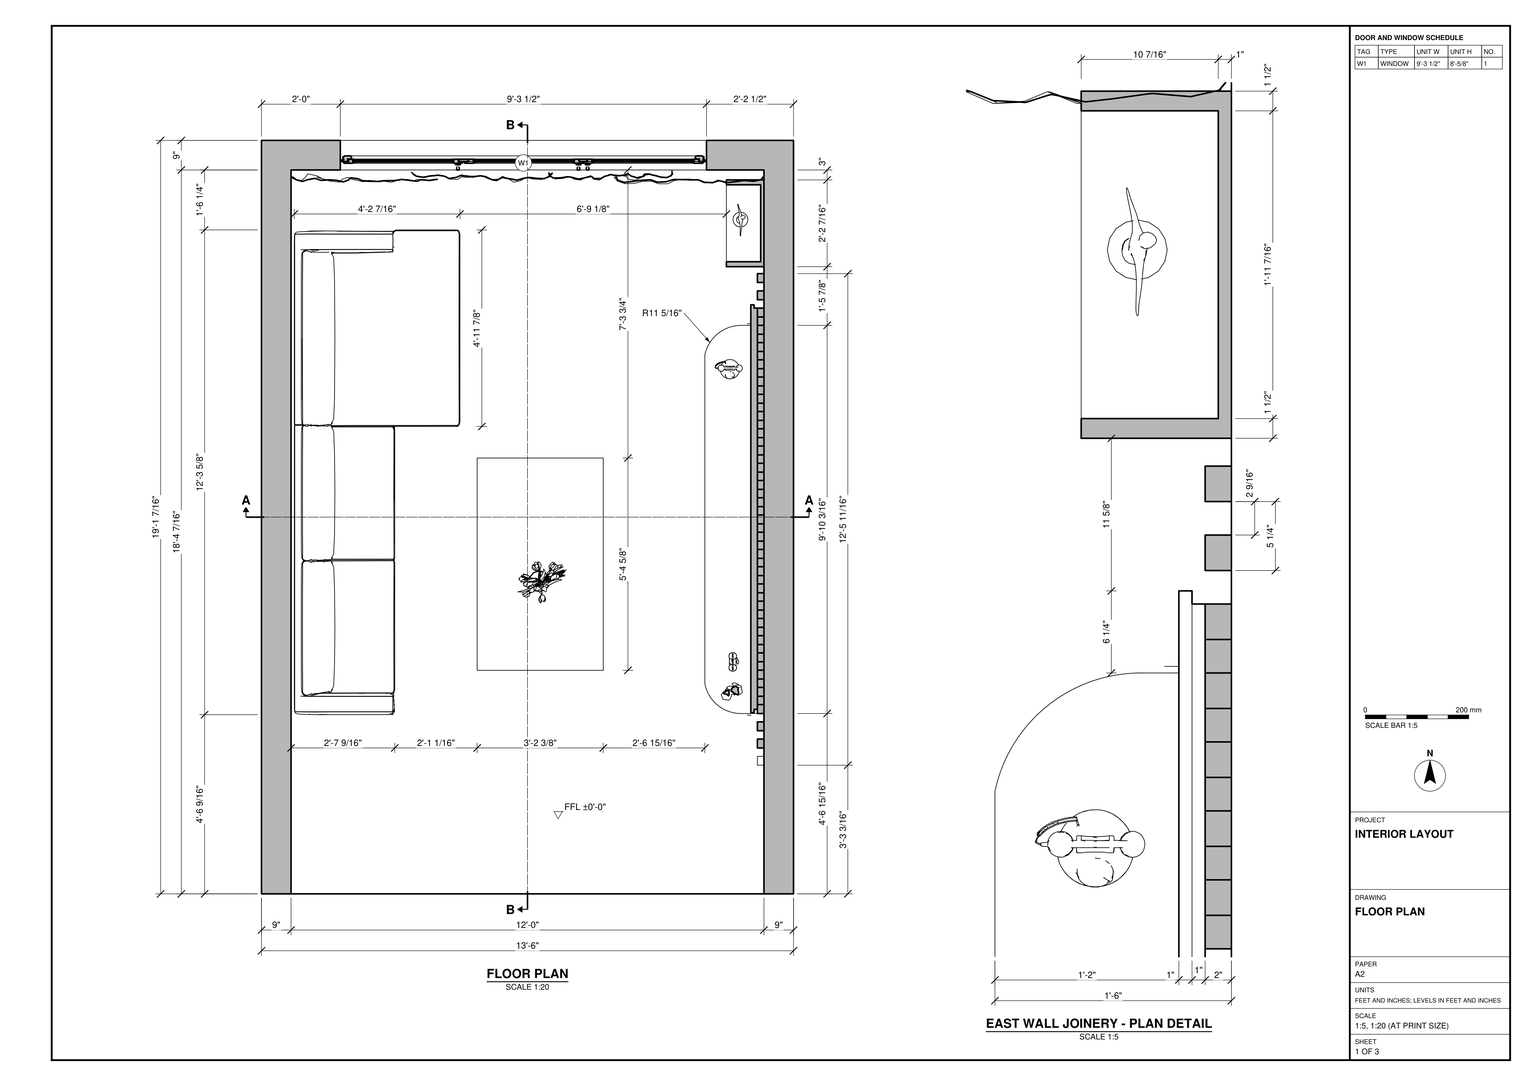
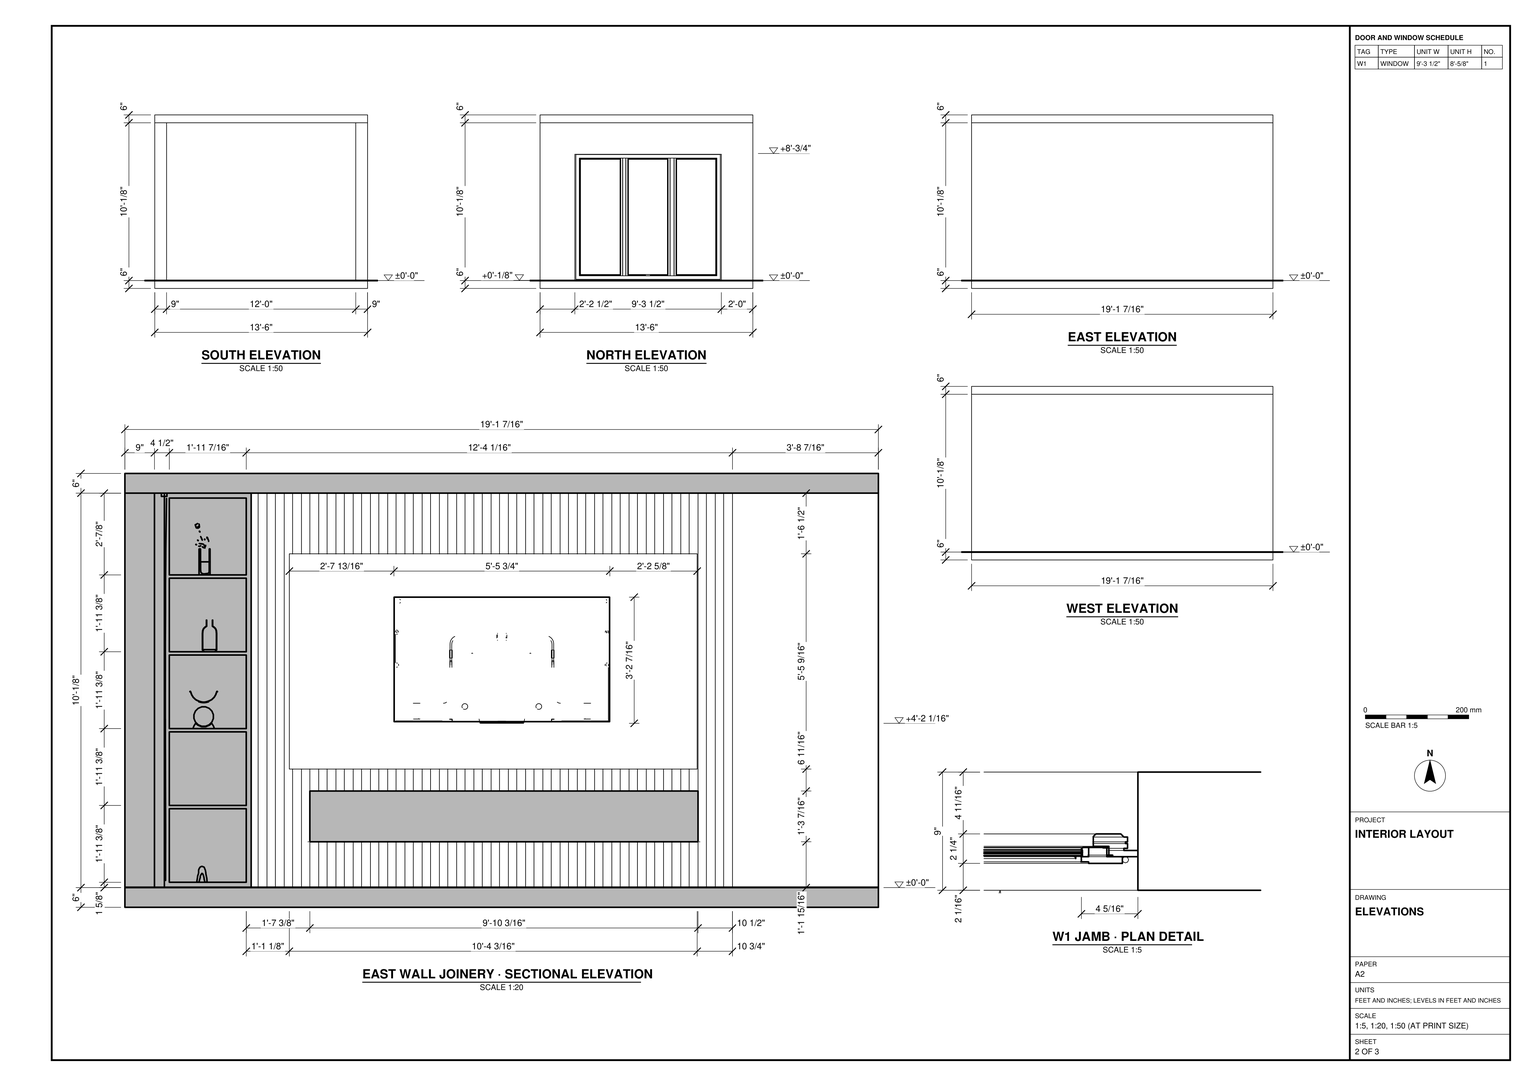
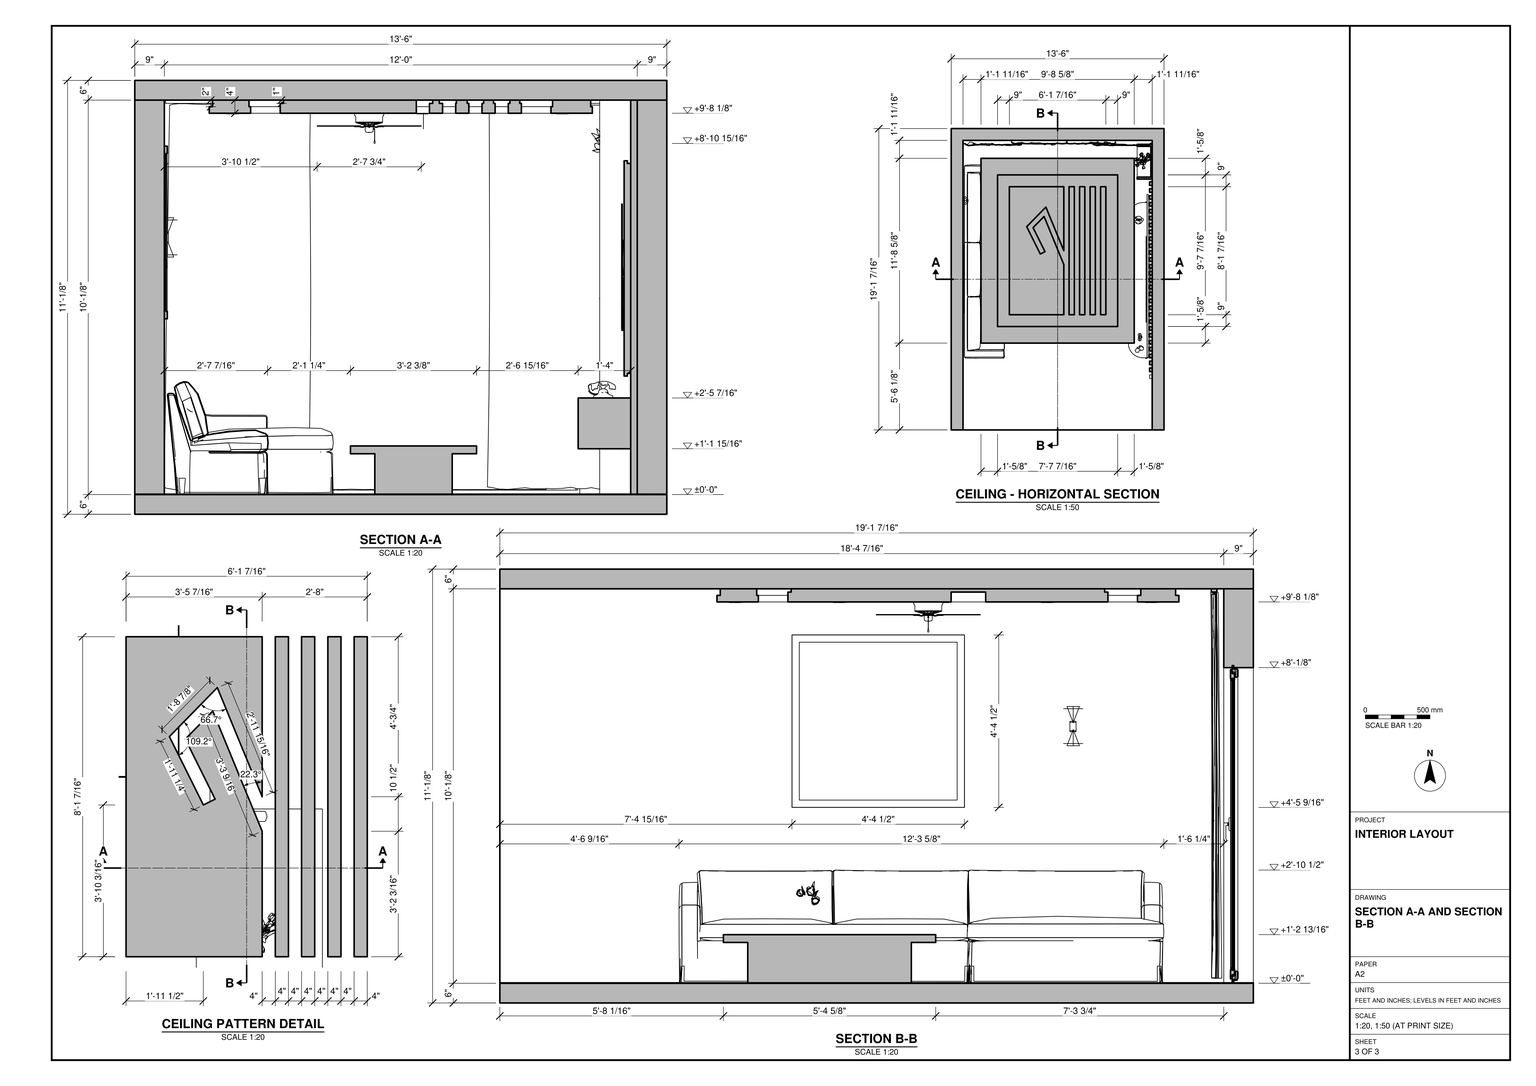
Build the living room in SketchUp from task_files/diagram_01.pdf. Work in feet and inches. Set the finished floor level to ±0'-0". The overall shell measures 13'-6" east to west, 19'-1 7/16" north to south and 11'-1/8" high. Model the 9" walls on the west, north and east sides, leaving the south end open as drawn. Include the 6" floor slab and 6" roof slab. Fit the wide, three-panel window into the north wall at the offset shown in plan, with curtains on the room side.

Place the long sofa against the west wall with its chaise at the window end. Set the rectangular pedestal coffee table between the sofa and the east wall. Use the east wall plan detail and sectional elevation together to model the open shelving tower beside the window, the vertical slats, the raised television backing panel and the floating console with rounded ends. Above the seating area, reproduce the stepped rectangular ceiling surround, the solid panel and the parallel strips. Include the ceiling fan, wall light, framed wall piece and shelf and tabletop objects in their indicated positions. Decor and loose items may be any suitable library components, for example from 3D Warehouse.

Keep the walls, slabs and each furniture or joinery piece in separate groups or components, and use components for repeated parts. Save one SketchUp model as output_files/living_room_with_media_joinery_and_patterned_ceiling.skp.

# SketchUp Ruby script. Lengths in inches.
U = 1.inch
M = Sketchup.active_model
def pt(a) = Geom::Point3d.new(a.map { |v| v * U })
def face(e, loops, mat)
  f = e.add_face(loops[0].map { |a| pt(a) })
  loops[1..].each { |l| e.add_face(l.map { |a| pt(a) }).erase! }
  f.material = f.back_material = mat if mat
  f
end
# faces: each face lists its corners as indices into pts; further lists are holes
def faces(e, pts, list, mat = nil) = list.each { |f| face(e, (f[0].is_a?(Array) ? f : [f]).map { |l| l.map { |i| pts[i] } }, mat) }
# xy, xz, yz: faces in a plane at the given z, y or x. An outline is a flat list of corners, or four numbers for a rectangle; further outlines are holes
def ring(l) = l.size == 4 ? [[l[0], l[1]], [l[2], l[1]], [l[2], l[3]], [l[0], l[3]]] : l.each_slice(2).to_a
def flat(e, list, mat, &to3) = list.each { |f| face(e, (f[0].is_a?(Array) ? f : [f]).map { |l| ring(l).map { |u, v| to3.(u, v) } }, mat) }
def xy(e, z, list, mat = nil) = flat(e, list, mat) { |x, y| [x, y, z] }
def xz(e, y, list, mat = nil) = flat(e, list, mat) { |x, z| [x, y, z] }
def yz(e, x, list, mat = nil) = flat(e, list, mat) { |y, z| [x, y, z] }
def lines(e, pts, list) = list.each { |a, b| e.add_line(pt(pts[a]), pt(pts[b])) }
# prism: a flat outline (further loops are holes) pulled along v
def prism(e, loops, v, mat = nil)
  f = face(e, loops, mat); d = Geom::Vector3d.new(v.map { |x| x * U })
  f.pushpull(f.normal.samedirection?(d) ? d.length : -d.length)
end
def box(e, o, s, mat = nil) = prism(e, [[o, [o[0] + s[0], o[1], o[2]], [o[0] + s[0], o[1] + s[1], o[2]], [o[0], o[1] + s[1], o[2]]]], [0, 0, s[2]], mat)
def at(x, y, z, deg = 0) = Geom::Transformation.translation(pt([x, y, z])) * Geom::Transformation.rotation(ORIGIN, Z_AXIS, deg.degrees)
def axes(o, x, y, z) = Geom::Transformation.new([*x, 0, *y, 0, *z, 0, *pt(o).to_a, 1])
def part(name) = M.definitions.add(name)
# library, detail: a bought-in or finely detailed component or shape, given as its bounding box
def library(name, o, s) = part(name).tap { |d| box(d.entities, o, s) }
def detail(e, o, s) = box(e.add_group.entities, o, s)
def put(e, d, t, mat = nil) = e.add_instance(d, t).tap { |i| i.material = mat if mat }
def group(e, t, mat = nil) = e.add_group.tap { |g| g.transformation = t; g.material = mat if mat }.entities
root = M.entities
M.materials.add("0209 AP 9428 SKY PINK1").color = [242, 235, 232]
M.materials.add("Emissive").color = [229, 231, 199]
M.materials.add("Generic").color = [255, 255, 255]
M.materials.add("Marble White 100cm").color = [255, 255, 255]
M.materials.add("Marble White 100cm\#2").color = [170, 170, 170]
M.materials.add("Marble White SSS 100cm\#2").color = [237, 237, 237]
M.materials.add("[Color B01]").color = [127, 96, 73]
M.materials.add("[Wood Board Cork]").color = [215, 201, 115]
M.materials.add("[Wood Veneer 01]").color = [120, 70, 37]
c1 = library("Window 46-13",[-55.59,-2.15,0],[111.18,4.3,92.91])
c2 = library("Curtains 001",[-91.88,-6.87,0.16],[183.71,15.03,109.46])
c3 = library("Fan 90-20",[-15.86,-15.86,-9.19],[31.73,31.72,9.19])
c4 = library("Vera Skirted Sofa with Chaise",[-47.18,-31.47,0.01],[94.62,63.06,34.48])
c5 = library("Phone 114 024",[-4.18,-2.9375,0],[8.35,5.89,5.09])
c6 = library("Alarm Clock 114 007",[-2.86,-1.17,0.01],[5.71,2.99,7.86])
c7 = library("Vase 193 006",[-6.57,-6.63,0],[14.76,12.62,17.43])
c8 = library("Tlon Light 450 Ceiling 152 006",[-8.86,-8.86,-3.78],[17.72,17.72,3.56])
c9 = library("Vase Roses Red 63-02",[-2.39,-2.73,0.01],[6.39,5.25,18.18])
c10 = library("Decorative Deer 209 004",[-1.58,-4.16,0],[3.36,7.25,10.63])
c11 = library("Scale 134 003",[-4.74,-4.74,0],[9.48,9.48,11.36])
c12 = library("Sculpture 108-23",[-12.84,-6.01,0],[25.68,12.02,38.36])
c13 = library("Vase 011",[-2.21,-2.21,0],[4.42,4.42,9.65])
c14 = library("Wall Light",[76.53,-3.84,-10.72],[14.73,32.02,29.93])
c15 = library("tv 56",[8.89,0,17.42],[39.61,3.79,23.15])
c16 = library("Group\#4",[-0.5,-0.5,-0.1],[2,24.43,0.2])
c17 = library("Group\#5",[-0.5,-0.5,-0.1],[2,24.43,0.2])
c18 = library("Group\#6",[-0.5,-0.5,-0.1],[2,24.43,0.2])
c19 = library("Group\#7",[-0.5,-0.5,-0.1],[2,24.43,0.2])
c20 = library("Group\#8",[-0.5,-0.5,-0.1],[2,24.43,0.2])
c21 = library("Group\#9",[-2,-147,0],[2,149.7,120])
c22 = library("Group\#10",[-0.5,-0.5,-0.1],[6,119.2,0.2])
xy(root,-0.125,[[0,67.4375,0,229.4375,162,229.4375,162,67.4375,153,67.4375,153,220.4375,9,220.4375,9,67.4375],[73.087,75.485,96.649,125.297]])
xy(root,0,[[0,0,9,67.4375],[153,0,162,67.4375],[0,67.4375,0,229.4375,24,229.4375,24,220.4375,9,220.4375,9,67.4375],[153,67.4375,153,220.4375,135.505,220.4375,135.505,229.4375,162,229.4375,162,67.4375],[141.5625,190.99,153,217.416],
  [24,220.4375,135.505,229.4375]])
xy(root,0,[[9,0,9,220.4375,153,220.4375,153,217.416,141.5625,217.416,141.5625,190.99,153,190.99,153,0]],"Marble White 100cm\#2")
xy(root,1.5,[[141.5625,192.489,152,215.916]],"[Wood Veneer 01]")
xy(root,12.3125,[[[65.669,68.067,104.067,132.715],[73.087,75.485,96.649,125.297]]],"Marble White SSS 100cm\#2")
xy(root,14.6875,[[65.669,68.067,104.067,132.715]],"Marble White SSS 100cm\#2")
xy(root,23.9,[[141.5625,192.489,151,215.916]],"[Wood Veneer 01]")
xy(root,24.9,[[141.5625,192.489,152,215.916]],"[Wood Veneer 01]")
xy(root,35.971,[[149,55.184,150,179.372]],"Marble White SSS 100cm\#2")
xy(root,36.781,[[150,56.184,151,178.372]],"Emissive")
xy(root,47.3,[[141.5625,192.489,151,215.916]],"[Wood Veneer 01]")
xy(root,48.3,[[141.5625,192.489,152,215.916]],"[Wood Veneer 01]")
xy(root,53.421,[[9,88.935,9.9,141.498]],"[Wood Veneer 01]")
xy(root,55.666,[[9.5,91.18,9.9,139.253]],"[Wood Veneer 01]")
xy(root,70.7,[[141.5625,192.489,151,215.916]],"[Wood Veneer 01]")
xy(root,71.7,[[141.5625,192.489,152,215.916]],"[Wood Veneer 01]")
xy(root,94.1,[[141.5625,192.489,151,215.916]],"[Wood Veneer 01]")
xy(root,95.1,[[141.5625,192.489,152,215.916]],"[Wood Veneer 01]")
xy(root,96,[[24,220.4375,135.505,229.4375]])
xy(root,100.72,[[150,56.184,151,178.372]],"Emissive")
xy(root,101.53,[[149,55.184,150,179.372]],"Marble White SSS 100cm\#2")
xy(root,103.739,[[9.5,91.18,9.9,139.253]])
xy(root,105.984,[[9,88.935,9.9,141.498]],"[Wood Veneer 01]")
xy(root,118.5,[[141.5625,192.489,151,215.916]])
xy(root,120,[[0,0,9,0,9,220.4375,153,220.4375,153,0,162,0,162,229.4375,0,229.4375],[9,0,153,0,153,190.99,141.5625,190.99,141.5625,217.416,153,217.416,153,220.4375,9,220.4375]])
xy(root,120,[[141.5625,190.99,153,217.416]],"[Wood Veneer 01]")
xz(root,0,[[0,0,9,120],[9,0,153,120],[153,0,162,120]])
xz(root,55.184,[[149,35.971,150,101.53]],"Marble White SSS 100cm\#2")
xz(root,56.184,[[150,36.781,151,100.72]],"Emissive")
xz(root,67.4375,[[0,-0.125,9,0],[153,-0.125,162,0]])
xz(root,68.067,[[65.669,12.3125,104.067,14.6875]],"Marble White SSS 100cm\#2")
xz(root,75.485,[[73.087,-0.125,96.649,12.3125]],"[Wood Veneer 01]")
xz(root,88.935,[[9,53.421,9.9,105.984]],"[Wood Veneer 01]")
xz(root,91.18,[[9.5,55.666,9.9,103.739]],"[Wood Veneer 01]")
xz(root,125.297,[[73.087,-0.125,96.649,12.3125]],"[Wood Veneer 01]")
xz(root,132.715,[[65.669,12.3125,104.067,14.6875]],"Marble White SSS 100cm\#2")
xz(root,139.253,[[9.5,55.666,9.9,103.739]],"[Wood Veneer 01]")
xz(root,141.498,[[9,53.421,9.9,105.984]],"[Wood Veneer 01]")
xz(root,178.372,[[150,36.781,151,100.72]],"Emissive")
xz(root,179.372,[[149,35.971,150,101.53]],"Marble White SSS 100cm\#2")
xz(root,190.99,[[141.5625,0,153,120]],"[Wood Veneer 01]")
xz(root,192.489,[[141.5625,1.5,152,23.9],[141.5625,24.9,152,47.3],[141.5625,48.3,152,70.7],[141.5625,71.7,152,94.1],[141.5625,95.1,152,118.5]],"[Wood Veneer 01]")
xz(root,215.916,[[141.5625,1.5,152,23.9],[141.5625,24.9,152,47.3],[141.5625,48.3,152,70.7],[141.5625,71.7,152,94.1],[141.5625,95.1,152,118.5]],"[Wood Veneer 01]")
xz(root,217.416,[[141.5625,0,153,120]],"[Wood Veneer 01]")
xz(root,220.4375,[[9,-0.125,153,0],[9,0,24,0,24,96,135.505,96,135.505,0,153,0,153,120,9,120]])
xz(root,229.4375,[[0,-0.125,24,0],[24,-0.125,135.505,0],[135.505,-0.125,162,0],[0,0,0,120,162,120,162,0,135.505,0,135.505,96,24,96,24,0]])
yz(root,0,[[67.4375,-0.125,229.4375,0],[0,0,229.4375,120]])
yz(root,9,[[67.4375,-0.125,220.4375,0],[88.935,53.421,141.498,105.984]])
yz(root,9,[[[0,0,220.4375,120],[88.935,53.421,141.498,105.984]]],"0209 AP 9428 SKY PINK1")
yz(root,9.5,[[91.18,55.666,139.253,103.739]],"[Color B01]")
yz(root,9.9,[[[88.935,53.421,141.498,105.984],[88.982,53.467,141.452,105.9375]],[[88.982,53.467,141.452,105.9375],[91.18,55.666,139.253,103.739]]],"[Wood Veneer 01]")
yz(root,24,[[220.4375,0,229.4375,96]])
yz(root,65.669,[[68.067,12.3125,132.715,14.6875]],"Marble White SSS 100cm\#2")
yz(root,73.087,[[75.485,-0.125,125.297,12.3125]],"[Wood Veneer 01]")
yz(root,96.649,[[75.485,-0.125,125.297,12.3125]],"[Wood Veneer 01]")
yz(root,104.067,[[68.067,12.3125,132.715,14.6875]],"Marble White SSS 100cm\#2")
yz(root,135.505,[[220.4375,0,229.4375,96]])
yz(root,141.5625,[[[190.99,0,217.416,120],[192.489,1.5,215.916,118.5]],[192.489,23.9,215.916,24.9],[192.489,47.3,215.916,48.3],[192.489,70.7,215.916,71.7],[192.489,94.1,215.916,95.1]],"[Wood Veneer 01]")
yz(root,149,[[55.184,35.971,179.372,101.53]],"Marble White SSS 100cm\#2")
yz(root,150,[[55.184,35.971,56.184,101.53],[56.184,35.971,179.372,36.781],[178.372,36.781,179.372,101.53],[56.184,100.72,178.372,101.53]],"Emissive")
yz(root,151,[[56.184,36.781,178.372,100.72]])
yz(root,152,[[192.489,1.5,215.916,23.9],[192.489,24.9,215.916,47.3],[192.489,48.3,215.916,70.7],[192.489,71.7,215.916,94.1],[192.489,95.1,215.916,118.5]],"[Wood Veneer 01]")
yz(root,153,[[67.4375,-0.125,220.4375,0],[0,0,186.171,120],[188.872,0,190.99,120],[190.99,0,217.416,120],[217.416,0,220.4375,120]])
yz(root,162,[[67.4375,-0.125,229.4375,0],[0,0,229.4375,120]])
p = [[146,173.122,13.834],[146,173.121,13.834]]
lines(root,p,[[0,1]])
detail(root,[135,54.92,13.83],[16,118.2,15.46])
put(root,c1,axes([79.75,222.58,0],[1.00292,0,0],[0,1,0],[0,0,1.04]))
put(root,c2,axes([81.02,218.15,1.22],[0.78383,0,0],[0,0.27996,0],[0,0,1.08359]))
put(root,c3,at(71.37,130.45,116))
put(root,c4,axes([35.25,128.16,-0.13],[0,1.56,0],[-0.8,0,0],[0,0,1]))
put(root,c5,at(142.24,159.76,29.29))
put(root,c6,at(143.48,70.64,29.28,-90))
put(root,c7,at(145.63,205.15,95.1))
put(root,c8,axes([29.89,71.7,116.54],[0.2,0,0],[0,0.2,0],[0,0,0.2]))
put(root,c9,at(142.4,61.73,29.28))
put(root,c10,at(145.87,205.98,1.5,-90))
put(root,c11,at(146.2,205.45,48.3,-90))
put(root,c12,axes([145.83,205.1875,24.9],[0,-0.38,0],[0.38,0,0],[0,0,0.38]))
put(root,c13,at(148.23,203.66,71.7))
put(root,c8,axes([29.89,103.375,116.54],[0.2,0,0],[0,0.2,0],[0,0,0.2]))
put(root,c8,axes([29.89,135.05,116.54],[0.2,0,0],[0,0.2,0],[0,0,0.2]))
put(root,c8,axes([29.89,166.72,116.54],[0.2,0,0],[0,0.2,0],[0,0,0.2]))
put(root,c8,axes([29.89,198.39,116.54],[0.2,0,0],[0,0.2,0],[0,0,0.2]))
put(root,c8,axes([68.71,71.7,116.54],[0.2,0,0],[0,0.2,0],[0,0,0.2]))
put(root,c8,axes([130.21,71.7,116.54],[0.2,0,0],[0,0.2,0],[0,0,0.2]))
put(root,c8,axes([130.21,103.89,116.54],[0.2,0,0],[0,0.2,0],[0,0,0.2]))
put(root,c8,axes([130.21,136.08,116.54],[0.2,0,0],[0,0.2,0],[0,0,0.2]))
put(root,c8,axes([130.21,168.27,116.54],[0.2,0,0],[0,0.2,0],[0,0,0.2]))
put(root,c8,axes([130.21,200.45,116.54],[0.2,0,0],[0,0.2,0],[0,0,0.2]))
put(root,c8,axes([87.58,200.45,116.54],[0.2,0,0],[0,0.2,0],[0,0,0.2]))
put(root,c14,axes([12.21,141.03,76.49],[0,0.4,0],[-0.184,0,0],[0,0,0.4]))
put(root,c7,at(84.61,95.19,14.6875))
put(root,c15,axes([149,67.02,20.98],[0,1.66,0],[-0.1826,0,0],[0,0,1.66]))
g1 = group(root,at(0,229.4375,-6.125),"Marble White 100cm")
box(g1,[0,-229.4375,0],[162,229.4375,6])
g2 = group(root,at(-329.75,43.4375,96),"[Wood Board Cork]")
xy(g2,20,[[[352.42,22.67,469.07,163.33],[365.02,35.27,456.47,150.73]]],"Generic")
xy(g2,20,[[374.02,44.27,374.02,141.73,415.47,141.73,415.47,93,401.81,126.24,387.22,111.31,397.57,90.49,401.15,92.27,392.07,110.55,400.42,119.1,411.77,91.48,415.47,82.48,415.47,44.27]],"[Wood Veneer 01]")
xy(g2,22,[[352.42,22.67,469.07,23.67],[352.42,23.67,353.42,163.33],[468.57,23.67,469.07,162.33],[364.52,34.77,365.02,150.73],[365.02,34.77,456.47,35.27],
  [456.47,34.77,456.97,150.73],[364.52,150.73,456.97,151.73],[353.42,162.33,469.07,163.33]],"Emissive")
xy(g2,23,[[415.47,82.48,411.77,91.48,400.42,119.1,392.07,110.55,401.15,92.27,397.57,90.49,387.22,111.31,401.81,126.24,415.47,93]])
xy(g2,23,[[374.02,44.27,415.47,45.27],[374.02,45.27,375.02,141.73],[375.02,140.73,415.47,141.73]],"Emissive")
xy(g2,24,[[375.02,45.27,415.47,140.73]])
xy(g2,24,[[[329.75,-43.4375,491.75,186],[353.42,23.67,468.57,162.33]],[[364.52,34.77,456.97,151.73],[375.02,45.27,415.47,140.73]]],"Generic")
xy(g2,30,[[329.75,-43.4375,491.75,186]])
xz(g2,-43.4375,[[329.75,24,491.75,30]],"Generic")
xz(g2,22.67,[[352.42,20,469.07,22]],"Generic")
xz(g2,23.67,[[353.42,22,468.57,24]],"Emissive")
xz(g2,34.77,[[364.52,22,456.97,24]],"Emissive")
xz(g2,35.27,[[365.02,20,456.47,22]],"Generic")
xz(g2,44.27,[[374.02,20,415.47,23]],"[Wood Veneer 01]")
xz(g2,45.27,[[375.02,23,415.47,24]],"Emissive")
xz(g2,140.73,[[375.02,23,415.47,24]],"Emissive")
xz(g2,141.73,[[374.02,20,415.47,23]])
xz(g2,150.73,[[365.02,20,456.47,22]],"Generic")
xz(g2,151.73,[[364.52,22,456.97,24]],"Emissive")
xz(g2,162.33,[[353.42,22,468.57,24]],"Emissive")
xz(g2,163.33,[[352.42,20,469.07,22]],"Generic")
xz(g2,186,[[329.75,24,491.75,30]],"Generic")
yz(g2,329.75,[[-43.4375,24,186,30]],"Generic")
yz(g2,352.42,[[22.67,20,163.33,22]],"Generic")
yz(g2,353.42,[[23.67,22,162.33,24]],"Emissive")
yz(g2,364.52,[[34.77,22,151.73,24]],"Emissive")
yz(g2,365.02,[[35.27,20,150.73,22]],"Generic")
yz(g2,374.02,[[44.27,20,141.73,23]])
yz(g2,375.02,[[45.27,23,140.73,24]],"Emissive")
yz(g2,415.47,[[44.27,20,82.48,23],[93,20,141.73,23]])
yz(g2,415.47,[[45.27,23,140.73,24]],"Emissive")
yz(g2,456.47,[[35.27,20,150.73,22]],"Generic")
yz(g2,456.97,[[34.77,22,151.73,24]],"Emissive")
yz(g2,468.57,[[23.67,22,162.33,24]],"Emissive")
yz(g2,469.07,[[22.67,20,163.33,22]],"Generic")
yz(g2,491.75,[[-43.4375,24,186,30]],"Generic")
p = [[415.47,82.48,20],[411.77,91.48,20],[411.77,91.48,23],[415.47,82.48,23],[397.57,90.49,20],[387.22,111.31,20],
  [387.22,111.31,23],[397.57,90.49,23],[401.15,92.27,20],[401.15,92.27,23],[400.42,119.1,20],[400.42,119.1,23],
  [392.07,110.55,20],[392.07,110.55,23],[401.81,126.24,20],[415.47,93,20],[415.47,93,23],[401.81,126.24,23]]
faces(g2,p,[[0,1,2,3],[4,5,6,7],[8,4,7,9],[1,10,11,2],[12,8,9,13],[14,15,16,17],[10,12,13,11],[5,14,17,6]],"Emissive")
g3 = group(g2,at(447.47,44.27,24))
xy(g3,-4,[[-28,0,-24,97.45],[-20,0,-16,97.45],[-12,0,-8,97.45],[-4,0,0,97.45]])
xy(g3,-1,[[-28,0,-25,1],[-25,0,-24,97.45],[-20,0,-16.5,0.1875],[-16.5,0,-16,97.45],[-12,0,-8,0.5],
  [-4,0,0,0.5],[-20,0.1875,-19.8125,97.45],[-12,0.5,-11.5,97.45],[-8.5,0.5,-8,97.45],[-4,0.5,-3.5,97.45],
  [-0.5,0.5,0,97.45],[-28,1,-27,97.45],[-27,96.45,-25,97.45],[-11.5,96.45,-8.5,97.45],[-3.5,96.45,-0.5,97.45],
  [-19.8125,97.26,-16.5,97.45]],"Emissive")
xy(g3,0,[[-19.8125,0.1875,-16.5,97.26],[-11.5,0.5,-8.5,96.45],[-3.5,0.5,-0.5,96.45],[-27,1,-25,96.45]])
xz(g3,0,[[-28,-4,-24,-1],[-20,-4,-16,-1],[-12,-4,-8,-1],[-4,-4,0,-1]])
xz(g3,0.1875,[[-19.8125,-1,-16.5,0]],"Emissive")
xz(g3,0.5,[[-11.5,-1,-8.5,0],[-3.5,-1,-0.5,0]],"Emissive")
xz(g3,1,[[-27,-1,-25,0]],"Emissive")
xz(g3,96.45,[[-27,-1,-25,0],[-11.5,-1,-8.5,0],[-3.5,-1,-0.5,0]],"Emissive")
xz(g3,97.26,[[-19.8125,-1,-16.5,0]],"Emissive")
xz(g3,97.45,[[-28,-4,-24,-1],[-20,-4,-16,-1],[-12,-4,-8,-1],[-4,-4,0,-1]])
yz(g3,-28,[[0,-4,97.45,-1]])
yz(g3,-27,[[1,-1,96.45,0]],"Emissive")
yz(g3,-25,[[1,-1,96.45,0]],"Emissive")
yz(g3,-24,[[0,-4,97.45,-1]])
yz(g3,-20,[[0,-4,97.45,-1]])
yz(g3,-19.8125,[[0.1875,-1,97.26,0]],"Emissive")
yz(g3,-16.5,[[0.1875,-1,97.26,0]],"Emissive")
yz(g3,-16,[[0,-4,97.45,-1]])
yz(g3,-12,[[0,-4,97.45,-1]])
yz(g3,-11.5,[[0.5,-1,96.45,0]],"Emissive")
yz(g3,-8.5,[[0.5,-1,96.45,0]],"Emissive")
yz(g3,-8,[[0,-4,97.45,-1]])
yz(g3,-4,[[0,-4,97.45,-1]])
yz(g3,-3.5,[[0.5,-1,96.45,0]],"Emissive")
yz(g3,-0.5,[[0.5,-1,96.45,0]],"Emissive")
yz(g3,0,[[0,-4,97.45,-1]])
put(root,c16,at(151,192.49,118.5))
put(root,c17,at(151,192.49,94.1))
put(root,c18,at(151,192.49,70.7))
put(root,c19,at(151,192.49,47.3))
put(root,c20,at(151,192.49,23.9))
put(root,c21,at(153,186.17,0))
put(root,c22,at(146,54.92,13.83),"[Wood Veneer 01]")
